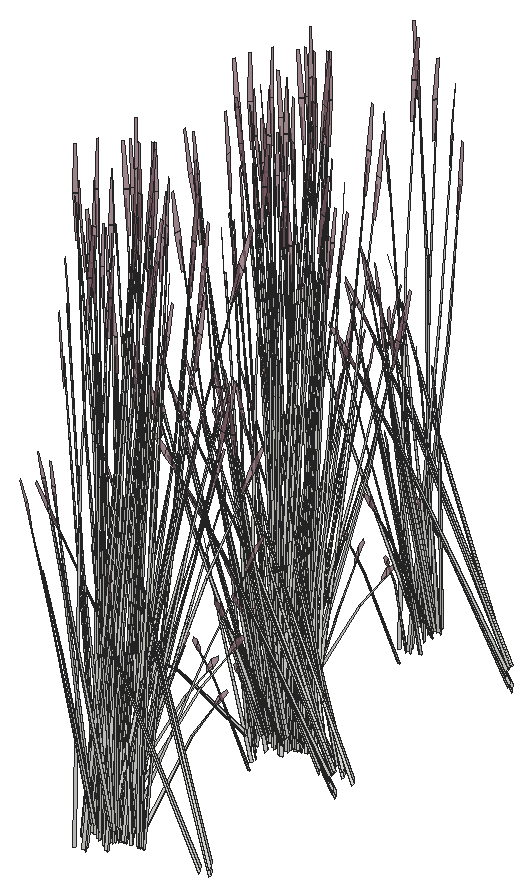
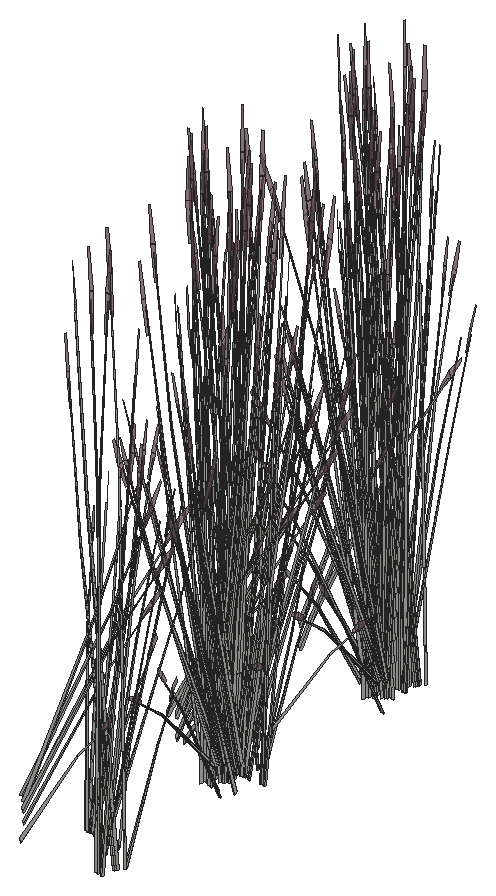
# SketchUp Ruby script. Lengths in inches.
U = 1.inch
M = Sketchup.active_model
def pt(a) = Geom::Point3d.new(a.map { |v| v * U })
def face(e, loops, mat)
  f = e.add_face(loops[0].map { |a| pt(a) })
  loops[1..].each { |l| e.add_face(l.map { |a| pt(a) }).erase! }
  f.material = f.back_material = mat if mat
  f
end
# faces: each face lists its corners as indices into pts; further lists are holes
def faces(e, pts, list, mat = nil) = list.each { |f| face(e, (f[0].is_a?(Array) ? f : [f]).map { |l| l.map { |i| pts[i] } }, mat) }
# xy, xz, yz: faces in a plane at the given z, y or x. An outline is a flat list of corners, or four numbers for a rectangle; further outlines are holes
def ring(l) = l.size == 4 ? [[l[0], l[1]], [l[2], l[1]], [l[2], l[3]], [l[0], l[3]]] : l.each_slice(2).to_a
def flat(e, list, mat, &to3) = list.each { |f| face(e, (f[0].is_a?(Array) ? f : [f]).map { |l| ring(l).map { |u, v| to3.(u, v) } }, mat) }
def xy(e, z, list, mat = nil) = flat(e, list, mat) { |x, y| [x, y, z] }
def xz(e, y, list, mat = nil) = flat(e, list, mat) { |x, z| [x, y, z] }
def yz(e, x, list, mat = nil) = flat(e, list, mat) { |y, z| [x, y, z] }
def lines(e, pts, list) = list.each { |a, b| e.add_line(pt(pts[a]), pt(pts[b])) }
# prism: a flat outline (further loops are holes) pulled along v
def prism(e, loops, v, mat = nil)
  f = face(e, loops, mat); d = Geom::Vector3d.new(v.map { |x| x * U })
  f.pushpull(f.normal.samedirection?(d) ? d.length : -d.length)
end
def box(e, o, s, mat = nil) = prism(e, [[o, [o[0] + s[0], o[1], o[2]], [o[0] + s[0], o[1] + s[1], o[2]], [o[0], o[1] + s[1], o[2]]]], [0, 0, s[2]], mat)
def at(x, y, z, deg = 0) = Geom::Transformation.translation(pt([x, y, z])) * Geom::Transformation.rotation(ORIGIN, Z_AXIS, deg.degrees)
def axes(o, x, y, z) = Geom::Transformation.new([*x, 0, *y, 0, *z, 0, *pt(o).to_a, 1])
def part(name) = M.definitions.add(name)
# library, detail: a bought-in or finely detailed component or shape, given as its bounding box
def library(name, o, s) = part(name).tap { |d| box(d.entities, o, s) }
def detail(e, o, s) = box(e.add_group.entities, o, s)
def put(e, d, t, mat = nil) = e.add_instance(d, t).tap { |i| i.material = mat if mat }
def group(e, t, mat = nil) = e.add_group.tap { |g| g.transformation = t; g.material = mat if mat }.entities
root = M.entities
M.materials.add("LightPink_Translucent").color = [144, 107, 117]
M.materials["LightPink_Translucent"].alpha = 0.75
c1 = part("blade")
p = [[2.15,0.21,22],[0,0.17,0],[0.09,0.45,0],[2.18,0.31,22],[2.29,0.31,22],[0.38,0.45,0],
  [2.48,0.24,33],[2.49,0.24,33],[2.48,0.22,33]]
faces(c1.entities,p,[[0,1,2,3],[4,5,2,3],[6,3,4,7],[8,0,3,6]])
c2 = part("seeds")
p = [[0.3,-0.1,1.38],[-0.01,-0.03,1.59],[-0.01,-0.03,0.03],[0.14,-0.07,-0.07],[0.29,-0.03,3],[0.15,0.01,3.11]]
faces(c2.entities,p,[[0,1,2,3],[1,0,4,5]],"LightPink_Translucent")
c3 = part("blade with seeds")
put(c3.entities,c1,at(0,0,0))
put(c3.entities,c2,axes([2.4,0.25,30.99],[1.5799,-0.05474,1.17369],[-0.12525,1.92788,0.29478],[-0.07173,-0.02425,1.56792]))
put(root,c3,axes([493.63,144.02,3.93],[0.74868,0.15974,0.48003],[-0.25601,0.52518,0.3958],[-0.04499,-0.20653,0.9933]))
put(root,c3,axes([495.39,144.84,4.23],[-0.83505,-0.03027,-0.1216],[0.02282,-0.57322,-0.67495],[0.05801,-0.22077,1.02557]))
put(root,c3,axes([495.33,144.47,3.72],[0.5141,-0.32171,-0.35414],[0.48666,0.36734,0.4572],[0.07405,-0.18664,0.87481]))
put(root,c3,axes([493.83,143.98,3.92],[0.55987,-0.20767,0.0643],[0.27403,0.37869,0.50621],[-0.05407,-0.16693,0.77189]))
put(root,c3,axes([493.62,144.4,4.24],[-0.22906,0.4699,0.35414],[-0.66828,-0.13705,-0.4572],[-0.06128,-0.18919,0.87481]))
put(root,c3,axes([495.53,144.64,3.92],[0.62439,0.02847,0.0643],[-0.01712,0.42991,0.50621],[0.06534,-0.16468,0.77189]))
put(root,c3,axes([495.0625,144.93,4.24],[-0.5141,0.32171,0.35414],[-0.48666,-0.36734,-0.4572],[0.07405,-0.18664,0.87481]))
put(root,c3,axes([491.68,144.39,1.57],[-0.47504,-0.61229,0],[0.79476,-0.34146,-0.51607],[0.18101,-0.07777,1.63711]))
put(root,c3,axes([492.33,144.3,1.21],[0.7111,-0.30552,-0.49651],[0.42504,0.54784,0],[0.16196,-0.06958,1.57504]))
put(root,c3,axes([492.28,146.36,1.4],[0.36864,-0.55059,-0.44739],[0.76598,0.26498,0.21531],[0,-0.12692,1.43643]))
put(root,c3,axes([492.61,146.08,1.86],[-0.08854,-0.69723,-0.29095],[0.92215,-0.04216,-0.50002],[0.16238,-0.09287,1.59708]))
put(root,c3,axes([492.49,144.54,1.22],[0.70886,0.15119,-0.30978],[-0.17848,0.53243,0.30978],[0.1429,-0.0614,1.38974]))
put(root,c3,axes([504.28,144.33,3.07],[0.31515,-0.01384,1.71376],[-0.20907,0.5998,0.13857],[-0.44912,-0.0371,0.73262]))
put(root,c3,axes([492.73,146.63,1.625],[0.8561,0.29616,0.24065],[-0.41201,0.61537,0.50002],[0,-0.14185,1.60543]))
put(root,c3,axes([492.46,146.22,1.91],[-0.82508,0.03772,0.44739],[-0.07462,-0.62614,-0.21531],[0.14771,-0.06346,1.43643]))
put(root,c3,axes([492.43,146.44,1.55],[0.33034,0.68327,0.45755],[-0.94388,0.2376,0.17955],[0.01154,-0.12555,1.58856]))
put(root,c3,axes([492.26,146.98,1.91],[-0.36864,0.55059,0.44739],[-0.76598,-0.26498,-0.21531],[0,-0.12692,1.43643]))
put(root,c3,axes([493.62,146.5,1.4],[0,-0.70701,0],[0.95008,0,0],[0,0,1.79456]))
put(root,c3,axes([494.77,144.87,1.67],[-0.7111,-0.30552,0.49651],[0.42504,-0.54784,0],[0.16196,0.06958,1.57504]))
put(root,c3,axes([493.17,146.06,1.55],[-0.62999,0.55453,0.45755],[-0.74845,-0.4895,0.17955],[0.15188,-0.05534,1.58856]))
put(root,c3,axes([493.85,147.05,1.49],[-0.70674,-0.52593,-0.06131],[0.70717,-0.52625,0],[-0.02468,-0.01837,1.75571]))
put(root,c3,axes([492.07,145.14,1.67],[-0.21949,0.60727,0.17642],[-0.8032,-0.17185,0.35086],[0.13875,-0.00296,1.60407]))
put(root,c3,axes([493.75,145.82,1.81],[0.14658,-0.54532,0.1448],[0.71613,0.09466,-0.41347],[0.13033,0.05599,1.26744]))
put(root,c3,axes([493.44,145.96,1.91],[-0.45644,-0.51287,0.44739],[0.69137,-0.36116,-0.21531],[0.14771,0.06346,1.43643]))
put(root,c3,axes([492,148.27,1.67],[0.81646,-0.16218,0.17642],[0.20161,0.60355,0.35086],[-0.07282,-0.08794,1.60407]))
put(root,c3,axes([494.26,146.66,1.4],[0.85008,0,0],[0,0.63259,0],[0,0,1.78407]))
put(root,c3,axes([494.5,145.18,1.67],[-0.81646,0.16218,0.17642],[-0.20161,-0.60355,0.35086],[0.07282,0.08794,1.60407]))
put(root,c3,axes([493.99,146.34,1.57],[-0.96033,-0.12874,0.49198],[0.19544,-0.7271,0.19306],[0.14034,0.07021,1.70813]))
put(root,c3,axes([493.22,148.13,1.4],[-0.24791,-0.5268,0],[0.70791,-0.18448,0],[0,0,1.54371]))
put(root,c3,axes([494.15,148.06,1.38],[0.79769,-0.20732,-0.19198],[0.2803,0.59721,0.00008],[0.08805,-0.02292,1.73897]))
put(root,c3,axes([494.43,148.31,1.67],[0.21949,-0.60727,0.17642],[0.8032,0.17185,0.35086],[-0.13875,0.00296,1.60407]))
put(root,c3,axes([494.24,146.93,1.41],[0.53038,0.39469,0],[-0.53038,0.39469,0],[0,0,1.69266]))
put(root,c3,axes([495.68,146.76,1.67],[-0.59697,-0.44509,0.17642],[0.60159,-0.4317,0.35086],[-0.06593,0.0909,1.60407]))
put(root,c3,axes([504.41,145.38,3.07],[0.26363,-0.12925,1.71376],[0.22195,0.59723,0.13857],[-0.41388,0.13498,0.73262]))
put(root,c3,axes([493.05,148.37,1.39],[-0.76598,-0.27433,0],[0.36864,-0.57001,0],[0,0,1.62707]))
put(root,c3,axes([494.24,146.47,1.91],[0.36864,-0.55059,0.44739],[0.76598,0.26498,-0.21531],[0,0.12692,1.43643]))
put(root,c3,axes([494.09,146.78,1.48],[0,0.70667,-0.05637],[-0.95008,0,0],[0,0.02221,1.79368]))
put(root,c3,axes([494.16,146.28,1.4],[0.45644,0.51287,-0.44739],[-0.69137,0.36116,0.21531],[0.14771,0.06346,1.43643]))
put(root,c3,axes([503.59,146.4,1.78],[0.26405,0.05016,1.43002],[0.17019,0.51235,-0.30754],[-0.35868,0.0959,0.61141]))
put(root,c3,axes([496.17,146.77,1.67],[0,-0.61104,0.49651],[0.85008,0,0],[0,0.13917,1.57504]))
put(root,c3,axes([494.04,147.23,1.91],[0.82508,-0.03772,0.44739],[0.07462,0.62614,-0.21531],[-0.14771,0.06346,1.43643]))
put(root,c3,axes([494.56,146.59,1.81],[0.70791,-0.1782,0.1448],[0.24791,0.50885,-0.41347],[0,0.11199,1.26744]))
put(root,c3,axes([493.92,148.38,1.4],[0.76598,0.27433,0],[-0.36864,0.57001,0],[0,0,1.74954]))
put(root,c3,axes([494.05,147.5,1.81],[0.56134,0.36712,0.1448],[-0.46823,0.41419,-0.41347],[-0.13033,0.05599,1.26744]))
put(root,c3,axes([494.65,148.63,1.67],[0.7111,-0.30552,0.49651],[0.42504,0.54784,0],[-0.16196,0.06958,1.57504]))
put(root,c3,axes([493.64,148.15,1.48],[0.33034,0.70197,-0.06012],[-0.94388,0.24598,0],[0.01154,0.02451,1.72173]))
put(root,c3,axes([496.37,147.23,1.39],[-0.94962,-0.00489,-0.04976],[0,-0.68292,0.49943],[-0.02984,0.15546,1.58352]))
put(root,c3,axes([494.3125,146.64,1.86],[0.85568,0.29155,-0.29095],[-0.41201,0.61537,-0.50002],[0.02689,0.15109,1.59708]))
put(root,c3,axes([496.17,147.33,1.22],[-0.53038,0.38124,-0.30978],[-0.53038,-0.38124,0.30978],[0,0.1228,1.38974]))
put(root,c3,axes([494.22,147.09,1.4],[-0.36864,0.55059,-0.44739],[-0.76598,-0.26498,0.21531],[0,0.12692,1.43643]))
put(root,c3,axes([494.01,148.86,4.24],[-0.11735,-0.49217,0.35414],[0.67083,-0.12996,-0.4572],[0.18018,0.14104,0.87481]))
put(root,c3,axes([494.24,148.67,1.52],[0.95122,0.19861,0.30756],[-0.23797,0.7099,-0.36492],[-0.15744,0.08885,1.64885]))
put(root,c3,axes([496.54,147.34,1.21],[0,0.61104,-0.49651],[-0.85008,0,0],[0,0.13917,1.57504]))
put(root,c3,axes([494.47,146.02,3.67],[-0.65655,-0.31748,1.38283],[0.69326,-0.49431,0.59665],[0.21183,0.29789,1.33663]))
put(root,c3,axes([495.46,148.61,1.96],[-0.4278,-0.1757,1.1486],[0.5524,-0.17852,0.84392],[0.14899,0.15122,0.25299]))
put(root,c3,axes([494.82,149.06,1.57],[0.47504,0.61229,0],[-0.79476,0.34146,-0.51607],[-0.18101,0.07777,1.63711]))
put(root,c3,axes([493.36,149.55,3.9],[0.00225,-0.07398,1.77383],[0.65113,-0.32638,-0.16761],[0.22617,0.1165,0.31391]))
put(root,c3,axes([494.66,147.26,1.29],[0.2786,0.55945,-0.69212],[-0.80253,0.20149,-0.18165],[0.03079,0.18945,1.52773]))
put(root,c3,axes([492.41,148.93,4.24],[0.22906,-0.4699,0.35414],[0.66828,0.13705,-0.4572],[0.06128,0.18919,0.87481]))
put(root,c3,axes([494.12,149.3,3.92],[-0.34533,0.38816,0.0643],[-0.49176,-0.22599,0.50621],[0.15898,0.12445,0.77189]))
put(root,c3,axes([493.31,150.61,4.84],[0.52505,-0.35054,-0.06488],[0.48109,0.38392,-0.29416],[0.03387,0.10878,0.97024]))
put(root,c3,axes([494.27,149.19,3.93],[-0.75571,0.14023,0.48003],[-0.13115,-0.55007,0.3958],[0.17773,0.16212,0.9933]))
put(root,c3,axes([493.93,148.42,1.78],[0.01341,-0.20255,1.43002],[0.64074,-0.22625,-0.30754],[0.1978,0.24243,0.61141]))
put(root,c3,axes([492.2,149.36,3.92],[-0.55987,0.20767,0.0643],[-0.27403,-0.37869,0.50621],[0.05407,0.16693,0.77189]))
put(root,c3,axes([492.1875,149.13,4.23],[0.74352,-0.28449,-0.1216],[0.36538,0.50492,-0.67495],[0.0981,0.21277,1.02557]))
put(root,c3,axes([492.4,149.32,4.26],[-0.74868,-0.15974,0.53283],[0.25601,-0.52518,0.43934],[0.04499,0.20653,1.10256]))
put(root,c3,axes([492.32,149.24,0.6875],[0.12297,-0.03325,1.76342],[0.73967,0.18301,-0.26939],[0.02163,0.20626,0.30037]))
put(root,c3,axes([492.82,149.11,3.875],[0.7469,0.15318,-0.51099],[-0.25601,0.52518,-0.3958],[0.06849,0.21144,0.97773]))
put(root,c3,axes([493.25,148.02,3.07],[-0.17368,-0.19618,1.71376],[0.80256,-0.16516,0.13857],[0.18139,0.30799,0.73262]))
put(root,c3,axes([492.48,149.43,3.72],[-0.22906,0.4699,-0.35414],[-0.66828,-0.13705,0.4572],[0.06128,0.18919,0.87481]))
put(root,c3,axes([492.55,149.01,4.17],[0.36264,0.49684,-0.71045],[-0.74649,0.27689,0.08574],[0.0848,0.24006,1.00501]))
put(root,c3,axes([492.01,150.26,3.91],[0.09631,0.0984,1.74944],[0.77725,0.03866,-0.27667],[0.07816,0.217,0.14031]))
put(root,c3,axes([503.24,162.28,3.07],[0.28223,0.10528,1.71376],[-0.58406,0.44165,0.13857],[-0.36402,-0.19924,0.73262]))
put(root,c3,axes([494.29,163.02,3.91],[-0.11621,-0.08567,1.74944],[-0.77555,0.05431,-0.27667],[-0.12378,-0.20491,0.14031]))
put(root,c3,axes([495.1,164.47,4.17],[-0.36264,-0.49684,-0.71045],[0.74649,-0.27689,0.08574],[-0.0848,-0.24006,1.00501]))
put(root,c3,axes([494.47,163.36,0.6875],[-0.12744,0.02202,1.76342],[-0.70477,-0.24781,-0.26939],[0.01183,-0.2067,0.30037]))
put(root,c3,axes([495.17,164.04,3.72],[0.22906,-0.4699,-0.35414],[0.66828,0.13705,0.4572],[-0.06128,-0.18919,0.87481]))
put(root,c3,axes([497.6,163.63,3.9],[-0.07716,0.04667,1.77383],[-0.75601,-0.15746,-0.16761],[-0.02737,-0.20368,0.31391]))
put(root,c3,axes([494.83,164.37,3.875],[-0.7469,-0.15318,-0.51099],[0.25601,-0.52518,-0.3958],[-0.06849,-0.21144,0.97773]))
put(root,c3,axes([495.29,163.05,1.96],[0.09747,0.35631,1.1486],[-0.54071,-0.19735,0.84392],[0.05818,-0.18244,0.25299]))
put(root,c3,axes([496.44,164.76,3.875],[-0.54391,-0.41056,-0.51099],[0.57458,-0.35956,-0.3958],[0.08276,-0.2086,0.97773]))
put(root,c3,axes([495.25,164.15,3.93],[0.74868,0.15974,0.48003],[-0.25601,0.52518,0.3958],[-0.04499,-0.20653,0.9933]))
put(root,c3,axes([495.47,164.34,4.23],[-0.74352,0.28449,-0.1216],[-0.36538,-0.50492,-0.67495],[-0.0981,-0.21277,1.02557]))
put(root,c3,axes([497.01,164.98,4.23],[-0.83505,-0.03027,-0.1216],[0.02282,-0.57322,-0.67495],[0.05801,-0.22077,1.02557]))
put(root,c3,axes([495.45,164.11,3.92],[0.55987,-0.20767,0.0643],[0.27403,0.37869,0.50621],[-0.05407,-0.16693,0.77189]))
put(root,c3,axes([502.97,162.84,1.78],[0.14835,0.17012,1.43002],[-0.34183,0.46242,-0.30754],[-0.351,-0.11053,0.61141]))
put(root,c3,axes([503.58,162.6875,4.17],[-0.75952,-0.01471,-0.71045],[0.05101,-0.61953,0.08574],[-0.32177,-0.06538,1.00501]))
put(root,c3,axes([493.42,166.33,1.29],[-0.31203,-0.62659,-0.69835],[0.89884,-0.22566,-0.18329],[-0.03449,-0.21218,1.54149]))
put(root,c3,axes([495.24,164.54,4.24],[-0.22906,0.4699,0.35414],[-0.66828,-0.13705,-0.4572],[-0.06128,-0.18919,0.87481]))
put(root,c3,axes([502.55,161.68,3.9],[0.05633,0.06098,1.77383],[-0.27155,0.54815,-0.16761],[-0.27501,0.00397,0.31391]))
put(root,c3,axes([496.68,165.07,4.24],[-0.5141,0.32171,0.35414],[-0.48666,-0.36734,-0.4572],[0.07405,-0.18664,0.87481]))
put(root,c3,axes([493.3,164.53,1.57],[-0.47504,-0.61229,0],[0.79476,-0.34146,-0.51607],[0.18101,-0.07777,1.63711]))
put(root,c3,axes([503.33,162.8125,3.875],[-0.55171,0.40476,-0.51099],[-0.48318,-0.42758,-0.3958],[-0.28031,-0.06159,0.97773]))
put(root,c3,axes([494.34,163.79,1.32],[-0.52505,0.35054,-0.03893],[-0.48109,-0.38392,-0.17649],[-0.03387,-0.10878,0.58215]))
put(root,c3,axes([502.64,163.25,3.07],[0.31515,-0.01384,1.71376],[-0.20907,0.5998,0.13857],[-0.44912,-0.0371,0.73262]))
put(root,c3,axes([491.58,166.25,1.21],[0,-0.61104,-0.49651],[0.85008,0,0],[0,-0.13917,1.57504]))
put(root,c3,axes([493.9,166.49,1.4],[0.36864,-0.55059,-0.44739],[0.76598,0.26498,0.21531],[0,-0.12692,1.43643]))
put(root,c3,axes([494.23,166.22,1.86],[-0.08854,-0.69723,-0.29095],[0.92215,-0.04216,-0.50002],[0.16238,-0.09287,1.59708]))
put(root,c3,axes([491.95,166.26,1.22],[0.53038,-0.38124,-0.30978],[0.53038,0.38124,0.30978],[0,-0.1228,1.38974]))
put(root,c3,axes([493.8,166.95,1.86],[-0.85568,-0.29155,-0.29095],[0.41201,-0.61537,-0.50002],[-0.02689,-0.15109,1.59708]))
put(root,c3,axes([502.44,163.98,0.6875],[0.01927,0.0963,1.76342],[-0.38846,0.5029,-0.26939],[-0.27592,-0.02535,0.30037]))
put(root,c3,axes([502.36,163.76,3.72],[-0.63144,-0.17046,-0.35414],[0.18417,-0.49731,0.4572],[-0.25423,0.0456,0.87481]))
put(root,c3,axes([494.35,166.77,1.625],[0.8561,0.29616,0.24065],[-0.41201,0.61537,0.50002],[0,-0.14185,1.60543]))
put(root,c3,axes([494.02,167.6,1.63],[0.20138,-0.72405,-0.23429],[0.95485,0.12621,0.51271],[-0.16685,-0.09999,1.5644]))
put(root,c3,axes([494.08,166.36,1.91],[-0.82508,0.03772,0.44739],[-0.07462,-0.62614,-0.21531],[0.14771,-0.06346,1.43643]))
put(root,c3,axes([504.29,163.68,2.53],[0.21597,-0.08839,1.77064],[0.07448,0.61717,0.13857],[-0.4678,0.08189,0.63284]))
put(root,c3,axes([491.95,166.8125,1.67],[0,0.61104,0.49651],[-0.85008,0,0],[0,-0.13917,1.57504]))
put(root,c3,axes([494.05,166.58,1.55],[0.33034,0.68327,0.45755],[-0.94388,0.2376,0.17955],[0.01154,-0.12555,1.58856]))
put(root,c3,axes([493.88,167.12,1.91],[-0.36864,0.55059,0.44739],[-0.76598,-0.26498,-0.21531],[0,-0.12692,1.43643]))
put(root,c3,axes([495.24,166.64,1.4],[0,-0.70701,0],[0.95008,0,0],[0,0,1.79456]))
put(root,c3,axes([501.96,164.09,3.91],[-0.12407,0.07933,1.74944],[0.01055,0.57963,-0.27667],[-0.2844,0.07538,0.14031]))
put(root,c3,axes([502.8,164.01,3.875],[-0.20584,0.55581,-0.51099],[-0.70573,-0.19051,-0.3958],[-0.28414,0.05097,0.97773]))
put(root,c3,axes([494.79,166.19,1.55],[-0.62999,0.55453,0.45755],[-0.74845,-0.4895,0.17955],[0.15188,-0.05534,1.58856]))
put(root,c3,axes([495.47,167.1875,1.49],[-0.70674,-0.52593,-0.06131],[0.70717,-0.52625,0],[-0.02468,-0.01837,1.75571]))
put(root,c3,axes([493.69,165.28,1.67],[-0.21949,0.60727,0.17642],[-0.8032,-0.17185,0.35086],[0.13875,-0.00296,1.60407]))
put(root,c3,axes([494.13,167.25,1.55],[0.96033,0.12874,0.45755],[-0.19544,0.7271,0.17955],[-0.14034,-0.07021,1.58856]))
put(root,c3,axes([495.0625,166.1,1.91],[-0.45644,-0.51287,0.44739],[0.69137,-0.36116,-0.21531],[0.14771,0.06346,1.43643]))
put(root,c3,axes([502.77,164.3,3.07],[0.26363,-0.12925,1.71376],[0.22195,0.59723,0.13857],[-0.41388,0.13498,0.73262]))
put(root,c3,axes([493.62,168.41,1.67],[0.81646,-0.16218,0.17642],[0.20161,0.60355,0.35086],[-0.07282,-0.08794,1.60407]))
put(root,c3,axes([495.88,166.8,1.4],[0.85008,0,0],[0,0.63259,0],[0,0,1.78407]))
put(root,c3,axes([496.12,165.3125,1.67],[-0.81646,0.16218,0.17642],[-0.20161,-0.60355,0.35086],[0.07282,0.08794,1.60407]))
put(root,c3,axes([501.95,165.32,1.78],[0.26405,0.05016,1.43002],[0.17019,0.51235,-0.30754],[-0.35868,0.0959,0.61141]))
put(root,c3,axes([500.59,164.68,3.9],[0.09697,0.01639,1.77383],[0.29997,0.53988,-0.16761],[-0.1985,0.1417,0.31391]))
put(root,c3,axes([495.61,166.48,1.57],[-0.96033,-0.12874,0.49198],[0.19544,-0.7271,0.19306],[0.14034,0.07021,1.70813]))
put(root,c3,axes([494.84,168.27,1.4],[-0.24791,-0.5268,0],[0.70791,-0.18448,0],[0,0,1.54371]))
put(root,c3,axes([494.37,167.77,1.81],[-0.14658,0.54532,0.1448],[-0.71613,-0.09466,-0.41347],[-0.13033,-0.05599,1.26744]))
put(root,c3,axes([496.05,168.45,1.67],[0.21949,-0.60727,0.17642],[0.8032,0.17185,0.35086],[-0.13875,0.00296,1.60407]))
put(root,c3,axes([495.86,167.07,1.41],[0.53038,0.39469,0],[-0.53038,0.39469,0],[0,0,1.69266]))
put(root,c3,axes([497.3,166.9,1.67],[-0.59697,-0.44509,0.17642],[0.60159,-0.4317,0.35086],[-0.06593,0.0909,1.60407]))
put(root,c3,axes([494.67,168.51,1.39],[-0.76598,-0.27433,0],[0.36864,-0.57001,0],[0,0,1.62707]))
put(root,c3,axes([495.86,166.61,1.91],[0.36864,-0.55059,0.44739],[0.76598,0.26498,-0.21531],[0,0.12692,1.43643]))
put(root,c3,axes([495.71,166.92,1.48],[0,0.70667,-0.05637],[-0.95008,0,0],[0,0.02221,1.79368]))
put(root,c3,axes([495.66,167.37,1.91],[0.82508,-0.03772,0.44739],[0.07462,0.62614,-0.21531],[-0.14771,0.06346,1.43643]))
put(root,c3,axes([496.18,166.73,1.81],[0.70791,-0.1782,0.1448],[0.24791,0.50885,-0.41347],[0,0.11199,1.26744]))
put(root,c3,axes([495.54,168.52,1.4],[0.76598,0.27433,0],[-0.36864,0.57001,0],[0,0,1.74954]))
put(root,c3,axes([495.84,169.125,1.39],[-0.46912,-0.61443,-0.05142],[0.79476,-0.34146,0.51607],[-0.19584,0.0585,1.6363]))
put(root,c3,axes([495.67,167.64,1.81],[0.56134,0.36712,0.1448],[-0.46823,0.41419,-0.41347],[-0.13033,0.05599,1.26744]))
put(root,c3,axes([496.27,168.77,1.67],[0.7111,-0.30552,0.49651],[0.42504,0.54784,0],[-0.16196,0.06958,1.57504]))
put(root,c3,axes([495.26,168.29,1.48],[0.33034,0.70197,-0.06012],[-0.94388,0.24598,0],[0.01154,0.02451,1.72173]))
put(root,c3,axes([495.625,169.05,1.22],[-0.70886,-0.15119,-0.30978],[0.17848,-0.53243,0.30978],[-0.1429,0.0614,1.38974]))
put(root,c3,axes([497.99,167.37,1.39],[-0.94962,-0.00489,-0.04976],[0,-0.68292,0.49943],[-0.02984,0.15546,1.58352]))
put(root,c3,axes([495.93,166.77,1.86],[0.85568,0.29155,-0.29095],[-0.41201,0.61537,-0.50002],[0.02689,0.15109,1.59708]))
put(root,c3,axes([497.79,167.47,1.22],[-0.53038,0.38124,-0.30978],[-0.53038,-0.38124,0.30978],[0,0.1228,1.38974]))
put(root,c3,axes([495.51,167.5,1.86],[0.08854,0.69723,-0.29095],[-0.92215,0.04216,-0.50002],[-0.16238,0.09287,1.59708]))
put(root,c3,axes([495.84,167.23,1.4],[-0.36864,0.55059,-0.44739],[-0.76598,-0.26498,0.21531],[0,0.12692,1.43643]))
put(root,c3,axes([495.86,168.81,1.52],[0.95122,0.19861,0.30756],[-0.23797,0.7099,-0.36492],[-0.15744,0.08885,1.64885]))
put(root,c3,axes([495.79,169.29,1.21],[-0.7111,0.30552,-0.49651],[-0.42504,-0.54784,0],[-0.16196,0.06958,1.57504]))
put(root,c3,axes([492.59,168.54,4.24],[0.5141,-0.32171,0.35414],[0.48666,0.36734,-0.4572],[-0.07405,0.18664,0.87481]))
put(root,c3,axes([496.4375,169.19,1.57],[0.47504,0.61229,0],[-0.79476,0.34146,-0.51607],[-0.18101,0.07777,1.63711]))
put(root,c3,axes([496.03,166.77,2.03],[-0.02076,-0.57531,1.41272],[0.93937,0.14913,0.59816],[-0.22217,0.31481,1.3335]))
put(root,c3,axes([496.28,167.4,1.29],[0.2786,0.55945,-0.69212],[-0.80253,0.20149,-0.18165],[0.03079,0.18945,1.52773]))
put(root,c3,axes([494.03,169.07,4.24],[0.22906,-0.4699,0.35414],[0.66828,0.13705,-0.4572],[0.06128,0.18919,0.87481]))
put(root,c3,axes([494.93,170.75,4.84],[0.52505,-0.35054,-0.06488],[0.48109,0.38392,-0.29416],[0.03387,0.10878,0.97024]))
put(root,c3,axes([493.82,169.5,3.92],[-0.55987,0.20767,0.0643],[-0.27403,-0.37869,0.50621],[0.05407,0.16693,0.77189]))
put(root,c3,axes([492.26,168.63,4.59],[0.83505,0.03027,-0.13498],[-0.02282,0.57322,-0.74919],[-0.05801,0.22077,1.13838]))
put(root,c3,axes([493.81,169.27,4.23],[0.74352,-0.28449,-0.1216],[0.36538,0.50492,-0.67495],[0.0981,0.21277,1.02557]))
put(root,c3,axes([494.02,169.46,4.26],[-0.74868,-0.15974,0.53283],[0.25601,-0.52518,0.43934],[0.04499,0.20653,1.10256]))
put(root,c3,axes([493.94,169.38,0.6875],[0.12297,-0.03325,1.76342],[0.73967,0.18301,-0.26939],[0.02163,0.20626,0.30037]))
put(root,c3,axes([492.83,168.85,4.2],[0.54391,0.41056,-0.5672],[-0.57458,0.35956,-0.43934],[-0.08276,0.2086,1.08528]))
put(root,c3,axes([492.24,169.46,2.02],[0.69024,-0.1082,0.06507],[0.15868,0.43593,-0.86304],[-0.04376,0.22067,0.7736]))
put(root,c3,axes([494.44,169.25,3.875],[0.7469,0.15318,-0.51099],[-0.25601,0.52518,-0.3958],[0.06849,0.21144,0.97773]))
put(root,c3,axes([494.1,169.57,3.72],[-0.22906,0.4699,-0.35414],[-0.66828,-0.13705,0.4572],[0.06128,0.18919,0.87481]))
put(root,c3,axes([493.45,168.26,3.07],[-0.0186,-0.23452,1.71376],[0.80601,0.15558,0.13857],[-0.04985,0.33422,0.73262]))
put(root,c3,axes([494.17,169.15,4.17],[0.36264,0.49684,-0.71045],[-0.74649,0.27689,0.08574],[0.0848,0.24006,1.00501]))
put(root,c3,axes([493.63,170.4,3.91],[0.09631,0.0984,1.74944],[0.77725,0.03866,-0.27667],[0.07816,0.217,0.14031]))
put(root,c3,axes([494.53,184.97,1.78],[-0.21597,0.12368,1.43002],[-0.64681,-0.21647,-0.30754],[0.1199,-0.26922,0.61141]))
put(root,c3,axes([493.55,185.4,4.17],[-0.36264,-0.49684,-0.71045],[0.74649,-0.27689,0.08574],[-0.0848,-0.24006,1.00501]))
put(root,c3,axes([492.92,184.3,0.6875],[-0.12744,0.02202,1.76342],[-0.70477,-0.24781,-0.26939],[0.01183,-0.2067,0.30037]))
put(root,c3,axes([495.06,185.88,4.17],[0.01977,-0.56521,-0.71045],[0.83252,0.03796,0.08574],[0.08786,-0.23945,1.00501]))
put(root,c3,axes([493.62,184.98,3.72],[0.22906,-0.4699,-0.35414],[0.66828,0.13705,0.4572],[-0.06128,-0.18919,0.87481]))
put(root,c3,axes([496.05,184.5625,3.9],[-0.07716,0.04667,1.77383],[-0.75601,-0.15746,-0.16761],[-0.02737,-0.20368,0.31391]))
put(root,c3,axes([503.47,184.38,3.07],[0.28223,0.10528,1.71376],[-0.58406,0.44165,0.13857],[-0.36402,-0.19924,0.73262]))
put(root,c3,axes([493.74,183.98,1.96],[0.09747,0.35631,1.1486],[-0.54071,-0.19735,0.84392],[0.05818,-0.18244,0.25299]))
put(root,c3,axes([494.89,185.7,3.875],[-0.54391,-0.41056,-0.51099],[0.57458,-0.35956,-0.3958],[0.08276,-0.2086,0.97773]))
put(root,c3,axes([493.7,185.08,3.93],[0.74868,0.15974,0.48003],[-0.25601,0.52518,0.3958],[-0.04499,-0.20653,0.9933]))
put(root,c3,axes([495.46,185.91,4.23],[-0.83505,-0.03027,-0.1216],[0.02282,-0.57322,-0.67495],[0.05801,-0.22077,1.02557]))
put(root,c3,axes([495.4,185.54,3.72],[0.5141,-0.32171,-0.35414],[0.48666,0.36734,0.4572],[0.07405,-0.18664,0.87481]))
put(root,c3,axes([493.9,185.04,3.92],[0.55987,-0.20767,0.0643],[0.27403,0.37869,0.50621],[-0.05407,-0.16693,0.77189]))
put(root,c3,axes([493.69,185.47,4.24],[-0.22906,0.4699,0.35414],[-0.66828,-0.13705,-0.4572],[-0.06128,-0.18919,0.87481]))
put(root,c3,axes([495.6,185.71,3.92],[0.62439,0.02847,0.0643],[-0.01712,0.42991,0.50621],[0.06534,-0.16468,0.77189]))
put(root,c3,axes([495.13,186,4.24],[-0.5141,0.32171,0.35414],[-0.48666,-0.36734,-0.4572],[0.07405,-0.18664,0.87481]))
put(root,c3,axes([491.75,185.46,1.57],[-0.47504,-0.61229,0],[0.79476,-0.34146,-0.51607],[0.18101,-0.07777,1.63711]))
put(root,c3,axes([503.2,184.9375,1.78],[0.14835,0.17012,1.43002],[-0.34183,0.46242,-0.30754],[-0.351,-0.11053,0.61141]))
put(root,c3,axes([503.82,184.79,4.17],[-0.75952,-0.01471,-0.71045],[0.05101,-0.61953,0.08574],[-0.32177,-0.06538,1.00501]))
put(root,c3,axes([492.39,185.37,1.21],[0.7111,-0.30552,-0.49651],[0.42504,0.54784,0],[0.16196,-0.06958,1.57504]))
put(root,c3,axes([503.5625,184.91,3.875],[-0.55171,0.40476,-0.51099],[-0.48318,-0.42758,-0.3958],[-0.28031,-0.06159,0.97773]))
put(root,c3,axes([492.35,187.43,1.4],[0.36864,-0.55059,-0.44739],[0.76598,0.26498,0.21531],[0,-0.12692,1.43643]))
put(root,c3,axes([492.68,187.15,1.86],[-0.08854,-0.69723,-0.29095],[0.92215,-0.04216,-0.50002],[0.16238,-0.09287,1.59708]))
put(root,c3,axes([502.875,185.34,3.07],[0.31515,-0.01384,1.71376],[-0.20907,0.5998,0.13857],[-0.44912,-0.0371,0.73262]))
put(root,c3,axes([492.5625,185.61,1.22],[0.70886,0.15119,-0.30978],[-0.17848,0.53243,0.30978],[0.1429,-0.0614,1.38974]))
put(root,c3,axes([492.8,187.7,1.625],[0.8561,0.29616,0.24065],[-0.41201,0.61537,0.50002],[0,-0.14185,1.60543]))
put(root,c3,axes([502.67,186.08,0.6875],[0.01927,0.0963,1.76342],[-0.38846,0.5029,-0.26939],[-0.27592,-0.02535,0.30037]))
